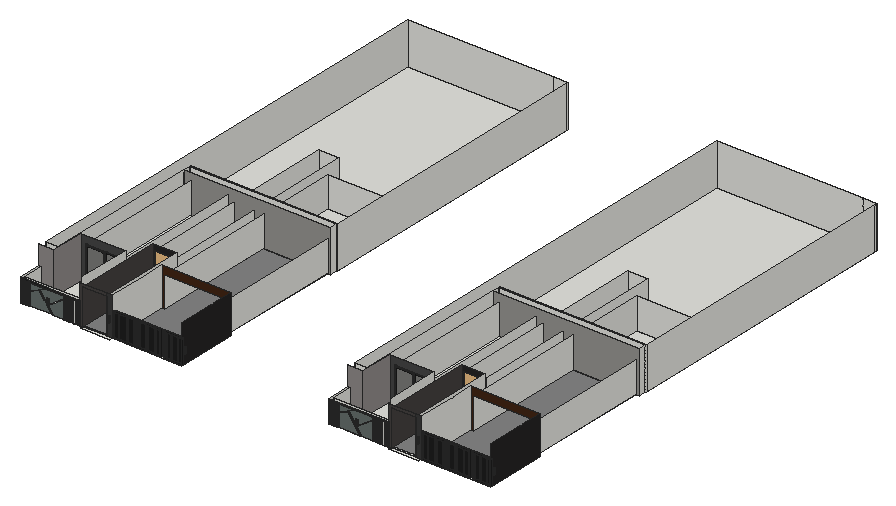
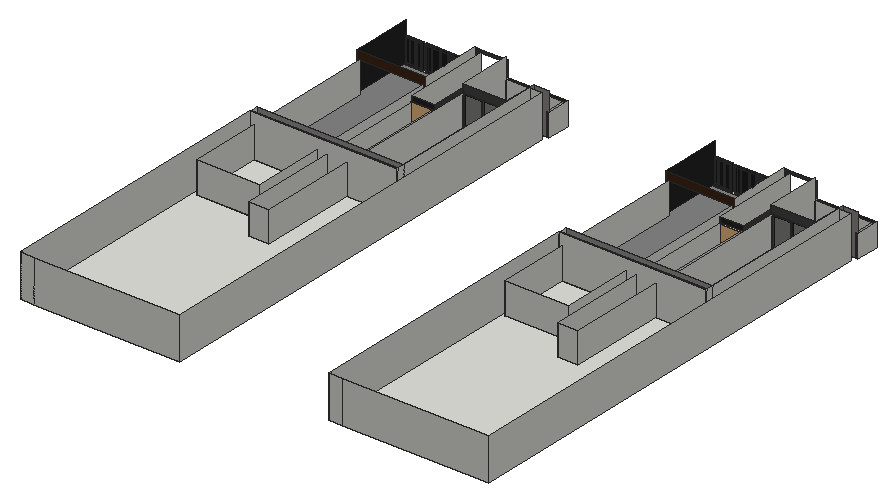
# SketchUp Ruby script. Lengths in inches.
U = 1.inch
M = Sketchup.active_model
def pt(a) = Geom::Point3d.new(a.map { |v| v * U })
def face(e, loops, mat)
  f = e.add_face(loops[0].map { |a| pt(a) })
  loops[1..].each { |l| e.add_face(l.map { |a| pt(a) }).erase! }
  f.material = f.back_material = mat if mat
  f
end
# faces: each face lists its corners as indices into pts; further lists are holes
def faces(e, pts, list, mat = nil) = list.each { |f| face(e, (f[0].is_a?(Array) ? f : [f]).map { |l| l.map { |i| pts[i] } }, mat) }
# xy, xz, yz: faces in a plane at the given z, y or x. An outline is a flat list of corners, or four numbers for a rectangle; further outlines are holes
def ring(l) = l.size == 4 ? [[l[0], l[1]], [l[2], l[1]], [l[2], l[3]], [l[0], l[3]]] : l.each_slice(2).to_a
def flat(e, list, mat, &to3) = list.each { |f| face(e, (f[0].is_a?(Array) ? f : [f]).map { |l| ring(l).map { |u, v| to3.(u, v) } }, mat) }
def xy(e, z, list, mat = nil) = flat(e, list, mat) { |x, y| [x, y, z] }
def xz(e, y, list, mat = nil) = flat(e, list, mat) { |x, z| [x, y, z] }
def yz(e, x, list, mat = nil) = flat(e, list, mat) { |y, z| [x, y, z] }
def lines(e, pts, list) = list.each { |a, b| e.add_line(pt(pts[a]), pt(pts[b])) }
# prism: a flat outline (further loops are holes) pulled along v
def prism(e, loops, v, mat = nil)
  f = face(e, loops, mat); d = Geom::Vector3d.new(v.map { |x| x * U })
  f.pushpull(f.normal.samedirection?(d) ? d.length : -d.length)
end
def box(e, o, s, mat = nil) = prism(e, [[o, [o[0] + s[0], o[1], o[2]], [o[0] + s[0], o[1] + s[1], o[2]], [o[0], o[1] + s[1], o[2]]]], [0, 0, s[2]], mat)
def at(x, y, z, deg = 0) = Geom::Transformation.translation(pt([x, y, z])) * Geom::Transformation.rotation(ORIGIN, Z_AXIS, deg.degrees)
def axes(o, x, y, z) = Geom::Transformation.new([*x, 0, *y, 0, *z, 0, *pt(o).to_a, 1])
def part(name) = M.definitions.add(name)
# library, detail: a bought-in or finely detailed component or shape, given as its bounding box
def library(name, o, s) = part(name).tap { |d| box(d.entities, o, s) }
def detail(e, o, s) = box(e.add_group.entities, o, s)
def put(e, d, t, mat = nil) = e.add_instance(d, t).tap { |i| i.material = mat if mat }
def group(e, t, mat = nil) = e.add_group.tap { |g| g.transformation = t; g.material = mat if mat }.entities
root = M.entities
M.materials.add("Glass_Tinted_Gray").color = [0, 0, 0]
M.materials["Glass_Tinted_Gray"].alpha = 0.125
M.materials.add("[0135_DarkGray]").color = [81, 81, 81]
M.materials.add("[Color M07]").color = [58, 58, 58]
M.materials.add("[Color M08]").color = [30, 30, 30]
M.materials.add("[Granite Dark Gray]").color = [38, 37, 37]
M.materials.add("[Granite Dark Gray]1").color = [69, 68, 68]
M.materials.add("[Granite Light Gray]").color = [149, 148, 144]
M.materials.add("[Granite Tile]1").color = [68, 65, 63]
M.materials.add("[Mirror 02]").color = [229, 229, 229]
M.materials.add("[Slate]").color = [102, 110, 108]
M.materials.add("[Stone Marble]").color = [143, 138, 136]
M.materials.add("[Terrazzo Light Blue]").color = [196, 214, 227]
M.materials.add("[Tile Grey]").color = [132, 132, 132]
M.materials.add("[Wood Veneer 01]").color = [66, 38, 20]
c1 = part("Group\#7")
xy(c1.entities,0,[[6,0,4.45,0.2,3,0.8,1.76,1.76,0.8,3,0.2,4.45,0,6,0.2,7.55,0.8,9,1.76,10.24,3,11.2,4.45,11.8,6,12,7.55,11.8,9,11.2,10.24,10.24,11.2,9,11.8,7.55,12,6,11.8,4.45,11.2,3,10.24,1.76,9,0.8,7.55,0.2]])
xy(c1.entities,37,[[6,0,7.55,0.2,9,0.8,10.24,1.76,11.2,3,11.8,4.45,12,6,11.8,7.55,11.2,9,10.24,10.24,9,11.2,7.55,11.8,6,12,4.45,11.8,3,11.2,1.76,10.24,0.8,9,0.2,7.55,0,6,0.2,4.45,0.8,3,1.76,1.76,3,0.8,4.45,0.2]],"[Granite Tile]1")
p = [[4.45,0.2,0],[6,0,0],[6,0,37],[4.45,0.2,37],[7.55,0.2,0],[7.55,0.2,37],
  [3,0.8,0],[3,0.8,37],[9,0.8,0],[9,0.8,37],[1.76,1.76,0],[1.76,1.76,37],
  [10.24,1.76,0],[10.24,1.76,37],[0.8,3,0],[0.8,3,37],[11.2,3,0],[11.2,3,37],
  [0.2,4.45,0],[0.2,4.45,37],[11.8,4.45,0],[11.8,4.45,37],[0,6,0],[0,6,37],
  [12,6,0],[12,6,37],[0.2,7.55,0],[0.2,7.55,37],[11.8,7.55,0],[11.8,7.55,37],
  [0.8,9,0],[0.8,9,37],[11.2,9,0],[11.2,9,37],[1.76,10.24,0],[1.76,10.24,37],
  [10.24,10.24,0],[10.24,10.24,37],[3,11.2,0],[3,11.2,37],[9,11.2,0],[9,11.2,37],
  [4.45,11.8,0],[4.45,11.8,37],[7.55,11.8,0],[7.55,11.8,37],[6,12,0],[6,12,37]]
faces(c1.entities,p,[[0,1,2,3],[1,4,5,2],[6,0,3,7],[4,8,9,5],[10,6,7,11],[8,12,13,9],[14,10,11,15],[12,16,17,13],
  [18,14,15,19],[16,20,21,17],[22,18,19,23],[20,24,25,21],[26,22,23,27],[24,28,29,25],[30,26,27,31],[28,32,33,29],
  [34,30,31,35],[32,36,37,33],[38,34,35,39],[36,40,41,37],[42,38,39,43],[40,44,45,41],[46,42,43,47],[44,46,47,45]],"[Granite Tile]1")
c2 = part("PENTEK_RP Fineline 50S_Sliding_DoorCase_E1")
box(c2.entities,[0,0,0],[1.51,3.66,99.27],"[0135_DarkGray]")
c3 = part("PENTEK_RP Fineline 50S_SlidingDooe_Case_E2")
box(c3.entities,[0,0,0],[96.25,3.66,1.51],"[0135_DarkGray]")
c4 = part("pentek_RP Fineline 50S_SlidingDoor_Case")
put(c4.entities,c2,at(97.76,0,0))
put(c4.entities,c3,at(1.51,0,0))
put(c4.entities,c2,at(0,0,0))
put(c4.entities,c3,at(1.51,0,97.76))
c5 = part("PENTEK_RP Fineline 50S_SlidingDoor_GlazingBead_2")
box(c5.entities,[0,0,0],[0.56,0.59,94.39],"[0135_DarkGray]")
c6 = part("PENTEK_RP Fineline 50S_SlidingDoor_Glass")
box(c6.entities,[0,0,0],[46.58,0.16,94.39],"Glass_Tinted_Gray")
c7 = part("PENTEK_RP Fineline 50S_SlidingDoor_GlazingBead")
box(c7.entities,[0,0,0],[45.47,0.59,0.56],"[0135_DarkGray]")
c8 = part("PENTEK_RP Fineline 50S_SlidingDoor_Leaf_E1")
xy(c8.entities,0,[[0,0,0.93,1.97],[0.93,1.57,1.49,1.97]],"[0135_DarkGray]")
xy(c8.entities,96.25,[[0,0,0.93,0,0.93,1.57,1.49,1.57,1.49,1.97,0,1.97]],"[0135_DarkGray]")
xz(c8.entities,0,[[0,0,0.93,96.25]],"[0135_DarkGray]")
xz(c8.entities,1.57,[[0.93,0,1.49,95.32],[0.93,95.32,1.49,96.25]],"[0135_DarkGray]")
xz(c8.entities,1.97,[[0,0,1.49,96.25]],"[0135_DarkGray]")
yz(c8.entities,0,[[0,0,1.97,96.25]],"[0135_DarkGray]")
yz(c8.entities,0.93,[[0,0,1.57,0.93],[0,0.93,1.57,95.32],[0,95.32,1.57,96.25]],"[0135_DarkGray]")
yz(c8.entities,1.49,[[1.57,0,1.97,95.32],[1.57,95.32,1.97,96.25]],"[0135_DarkGray]")
c9 = part("PENTEK_RP Fineline 50S_SlidingDoor_Leaf_E2")
xy(c9.entities,0,[[0,0,0,1.57,0.56,1.57,0.56,1.97,46.02,1.97,46.02,1.57,46.58,1.57,46.58,0]],"[0135_DarkGray]")
xy(c9.entities,0.93,[[0,0,46.58,1.57]],"[0135_DarkGray]")
xy(c9.entities,1.49,[[0.56,1.57,46.02,1.97]],"[0135_DarkGray]")
xz(c9.entities,0,[[0,0,46.58,0.93]],"[0135_DarkGray]")
xz(c9.entities,1.57,[[0,0,0.56,0.93],[46.02,0,46.58,0.93],[0.56,0.93,46.02,1.49]],"[0135_DarkGray]")
xz(c9.entities,1.97,[[0.56,0,46.02,1.49]],"[0135_DarkGray]")
yz(c9.entities,0,[[0,0,1.57,0.93]],"[0135_DarkGray]")
yz(c9.entities,0.56,[[1.57,0,1.97,0.93],[1.57,0.93,1.97,1.49]],"[0135_DarkGray]")
yz(c9.entities,46.02,[[1.57,0,1.97,0.93],[1.57,0.93,1.97,1.49]],"[0135_DarkGray]")
yz(c9.entities,46.58,[[0,0,1.57,0.93]],"[0135_DarkGray]")
c10 = part("PENTEK_RP Fineline S_SlidingDoor_Leaf1")
put(c10.entities,c5,at(0.93,0,0.93))
put(c10.entities,c5,at(46.96,0,0.93))
put(c10.entities,c6,at(1.49,1.42,0.93))
put(c10.entities,c7,at(1.49,0,0.93))
put(c10.entities,c6,at(1.49,0.59,0.93),"[Terrazzo Light Blue]")
put(c10.entities,c8,at(0,0,0))
put(c10.entities,c8,axes([48.44,0,0],[-1,0,0],[0,1,0],[0,0,1]))
put(c10.entities,c9,axes([0.93,0,96.25],[1,0,0],[0,1,0],[0,0,-1]))
put(c10.entities,c9,at(0.93,0,0))
put(c10.entities,c7,at(1.49,0,94.77))
c11 = part("PENTEK_RP Fineline 50S_SlidingDoor_Leaf2")
put(c11.entities,c6,at(1.49,1.42,0.93))
put(c11.entities,c7,at(1.49,0,94.77))
put(c11.entities,c5,at(46.96,0,0.93))
put(c11.entities,c6,at(1.49,0.59,0.93),"[Mirror 02]")
put(c11.entities,c5,at(0.93,0,0.93))
put(c11.entities,c8,at(0,0,0))
put(c11.entities,c8,axes([48.44,0,0],[-1,0,0],[0,1,0],[0,0,1]))
put(c11.entities,c7,at(1.49,0,0.93))
put(c11.entities,c9,axes([0.93,0,96.25],[1,0,0],[0,1,0],[0,0,-1]))
put(c11.entities,c9,at(0.93,0,0))
c12 = part("PENTEK - Slimmest Steel Sliding Door / Window\#1")
put(c12.entities,c4,at(0,-1.88,-0.09))
put(c12.entities,c10,at(1.51,-2.27,1.42))
put(c12.entities,c11,at(49.32,-0.3,1.42))
c13 = library("元件\#5",[-4.39,0,0],[5.37,35.83,90.55])
c14 = part("Group\#102")
g1 = group(c14.entities,at(0,0,0))
prism(g1,[[[0,3,72],[70.5,3,72],[70.5,3,0],[0,3,0]],[[67.5,3,3],[67.5,3,69],[3,3,69],[3,3,3]]],[0,-3,0])
c15 = part("Group\#135")
box(c15.entities,[0,0,0],[0.5,1,66])
c16 = part("Group\#148")
box(c16.entities,[0,-1,0],[5.5,1,66])
box(c16.entities,[50.84,-1,0],[13.66,1,66])
box(c16.entities,[28.06,-1,0],[22.28,1,66])
box(c16.entities,[24.66,-1,0],[2.9,1,66])
box(c16.entities,[6,-1,0],[18.16,1,66])
c17 = part("Component\#23")
g2 = group(c17.entities,at(70.5,0,0),"[Color M08]")
put(g2,c14,axes([70.5,0,0],[-1,0,0],[0,1,0],[0,0,1]))
g3 = group(g2,at(3,2,3))
g4 = group(g3,at(0,-1,0))
box(g4,[0,0,0],[5.5,1,66])
box(g4,[50.84,0,0],[13.66,1,66])
box(g4,[28.06,0,0],[22.28,1,66])
box(g4,[24.66,0,0],[2.9,1,66])
box(g4,[6,0,0],[18.16,1,66])
put(g3,c15,axes([50.34,0,0],[1,0,0],[0,-1,0],[0,0,1]))
put(g3,c15,axes([24.16,0,0],[1,0,0],[0,-1,0],[0,0,1]))
put(g3,c15,axes([27.56,0,0],[1,0,0],[0,-1,0],[0,0,1]))
put(g3,c15,axes([5.5,0,0],[1,0,0],[0,-1,0],[0,0,1]))
g5 = group(c17.entities,at(70.5,0,0),"[Color M08]")
put(g5,c14,at(-70.5,0,0))
g6 = group(g5,at(-3,2,3,-180))
put(g6,c16,at(0,1,0))
put(g6,c15,at(50.34,0,0))
put(g6,c15,at(24.16,0,0))
put(g6,c15,at(27.56,0,0))
put(g6,c15,at(5.5,0,0))
g7 = group(c17.entities,at(150,0,0),"[Color M08]")
put(g7,c14,axes([54,0,0],[-0.76596,0,0],[0,1,0],[0,0,1]))
g8 = group(g7,at(2.3,2,3))
put(g8,c16,axes([0,-1,0],[0.76596,0,0],[0,-1,0],[0,0,1]))
put(g8,c15,axes([38.55,0,0],[0.76596,0,0],[0,-1,0],[0,0,1]))
put(g8,c15,axes([18.5,0,0],[0.76596,0,0],[0,-1,0],[0,0,1]))
put(g8,c15,axes([21.11,0,0],[0.76596,0,0],[0,-1,0],[0,0,1]))
put(g8,c15,axes([4.22,0,0],[0.76596,0,0],[0,-1,0],[0,0,1]))
xy(root,8.5,[[2153.45,450,2237.65,458.5],[3032.2,450,3116.4,458.5],[1976.47,457.5625,1980.03,458.5],[1981.28,457.5625,1984.84,458.5],[1986.1,457.5625,1989.66,458.5],
  [1990.91,457.5625,1994.47,458.5],[1995.72,457.5625,1999.28,458.5],[2000.53,457.5625,2004.09,458.5],[2100.97,457.5625,2104.93,458.5],[2105.97,457.5625,2109.93,458.5],
  [2110.97,457.5625,2114.93,458.5],[2115.97,457.5625,2119.93,458.5],[2120.97,457.5625,2124.93,458.5],[2125.97,457.5625,2129.93,458.5],[2135.7,457.5625,2139.36,458.5],
  [2143.16,457.5625,2146.28,458.5],[2855.22,457.5625,2858.78,458.5],[2860.03,457.5625,2863.59,458.5],[2864.85,457.5625,2868.41,458.5],[2869.66,457.5625,2873.22,458.5],
  [2874.47,457.5625,2878.03,458.5],[2879.28,457.5625,2882.84,458.5],[2979.72,457.5625,2983.68,458.5],[2984.72,457.5625,2988.68,458.5],[2989.72,457.5625,2993.68,458.5],
  [2994.72,457.5625,2998.68,458.5],[2999.72,457.5625,3003.68,458.5],[3004.72,457.5625,3008.68,458.5],[3014.45,457.5625,3018.11,458.5],[3021.91,457.5625,3025.03,458.5],
  [1976.47,458.5,1976.47,523.18,1983.29,523.18,1983.29,465.32,2146.28,465.32,2146.28,458.5,2067.62,458.5,2067.62,461.375,2064.07,461.375,2064.07,458.5],[2064.07,458.5,2067.62,461.375],[2153.45,458.5,2221.2,465.32],[2238.79,458.5,2436.4,465.32],[2855.22,458.5,2855.22,523.18,2862.04,523.18,2862.04,465.32,3025.03,465.32,3025.03,458.5,2946.37,458.5,2946.37,461.375,2942.82,461.375,2942.82,458.5],
  [2942.82,458.5,2946.37,461.375],[3032.2,458.5,3099.95,465.32],[3117.54,458.5,3315.15,465.32],[1983.29,465.32,2146.28,465.32,2146.28,619.06,2020.16,619.06,2020.16,523.18,1983.29,523.18],[2862.04,465.32,3025.03,465.32,3025.03,619.06,2898.91,619.06,2898.91,523.18,2862.04,523.18],
  [1983.29,539.02,2019.03,539.02,2019.03,1010.9,2160.47,1010.9,2160.47,1288.43,2218.35,1288.43,2218.35,1010.9,2246.4,1010.9,2246.4,1213.68,2427.3,1213.68,2427.3,1010.9,2436.4,1010.9,2436.4,1828.81,1983.29,1828.81],[2862.04,539.02,2897.78,539.02,2897.78,1010.9,3039.22,1010.9,3039.22,1288.43,3097.1,1288.43,3097.1,1010.9,3125.15,1010.9,3125.15,1213.68,3306.05,1213.68,3306.05,1010.9,3315.15,1010.9,3315.15,1828.81,2862.04,1828.81],[2019.03,986.46,2160.47,1006.15],[2160.47,986.46,2218.35,1006.15],[2218.35,986.46,2246.4,1006.15],
  [2246.4,986.46,2427.3,1006.15],[2427.3,986.46,2436.4,1006.15],[2897.78,986.46,3039.22,1006.15],[3039.22,986.46,3097.1,1006.15],[3097.1,986.46,3125.15,1006.15],
  [3125.15,986.46,3306.05,1006.15],[3306.05,986.46,3315.15,1006.15],[2019.03,1006.15,2160.47,1010.9],[2160.47,1006.15,2218.35,1010.9],[2218.35,1006.15,2246.4,1010.9],
  [2246.4,1006.15,2427.3,1010.9],[2427.3,1006.15,2436.4,1010.9],[2897.78,1006.15,3039.22,1010.9],[3039.22,1006.15,3097.1,1010.9],[3097.1,1006.15,3125.15,1010.9],
  [3125.15,1006.15,3306.05,1010.9],[3306.05,1006.15,3315.15,1010.9],[2160.47,1010.9,2218.35,1288.43],[2246.4,1010.9,2427.3,1213.68],[3039.22,1010.9,3097.1,1288.43],
  [3125.15,1010.9,3306.05,1213.68]])
xy(root,8.5,[[2153.45,465.32,2221.2,465.32,2221.2,706.62,2218.35,706.62,2218.35,986.46,2160.47,986.46,2160.47,706.62,2153.45,706.62],[2238.79,465.32,2436.4,465.32,2436.4,633.06,2427.3,633.06,2427.3,986.46,2246.4,986.46,2246.4,633.06,2238.79,633.06],[3032.2,465.32,3099.95,465.32,3099.95,706.62,3097.1,706.62,3097.1,986.46,3039.22,986.46,3039.22,706.62,3032.2,706.62],[3117.54,465.32,3315.15,465.32,3315.15,633.06,3306.05,633.06,3306.05,986.46,3125.15,986.46,3125.15,633.06,3117.54,633.06]],"[Tile Grey]")
xy(root,20.01,[[2037.38,619.06,2142.51,1006.15],[2916.13,619.06,3021.26,1006.15]])
xy(root,68.78,[[1980.03,457.5625,1981.28,458.5],[1984.84,457.5625,1986.1,458.5],[1989.66,457.5625,1990.91,458.5],[1994.47,457.5625,1995.72,458.5],[1999.28,457.5625,2000.53,458.5],
  [2004.09,457.5625,2004.09,458.5,2047.85,458.5,2047.85,461.375,2050.98,461.375,2050.98,458.5,2100.97,458.5,2100.97,457.5625],[2104.93,457.5625,2105.97,458.5],[2109.93,457.5625,2110.97,458.5],[2114.93,457.5625,2115.97,458.5],[2119.93,457.5625,2120.97,458.5],
  [2124.93,457.5625,2125.97,458.5],[2129.93,457.5625,2135.7,458.5],[2139.36,457.5625,2143.16,458.5],[2858.78,457.5625,2860.03,458.5],[2863.59,457.5625,2864.85,458.5],
  [2868.41,457.5625,2869.66,458.5],[2873.22,457.5625,2874.47,458.5],[2878.03,457.5625,2879.28,458.5],[2882.84,457.5625,2882.84,458.5,2926.6,458.5,2926.6,461.375,2929.73,461.375,2929.73,458.5,2979.72,458.5,2979.72,457.5625],[2983.68,457.5625,2984.72,458.5],
  [2988.68,457.5625,2989.72,458.5],[2993.68,457.5625,2994.72,458.5],[2998.68,457.5625,2999.72,458.5],[3003.68,457.5625,3004.72,458.5],[3008.68,457.5625,3014.45,458.5],
  [3018.11,457.5625,3021.91,458.5]])
xz(root,457.5625,[[1976.47,8.5,1980.03,68.78],[1981.28,8.5,1984.84,68.78],[1986.1,8.5,1989.66,68.78],[1990.91,8.5,1994.47,68.78],[1995.72,8.5,1999.28,68.78],
  [2000.53,8.5,2004.09,68.78],[2100.97,8.5,2104.93,68.78],[2105.97,8.5,2109.93,68.78],[2110.97,8.5,2114.93,68.78],[2115.97,8.5,2119.93,68.78],
  [2120.97,8.5,2124.93,68.78],[2143.16,8.5,2146.28,68.78],[2855.22,8.5,2858.78,68.78],[2860.03,8.5,2863.59,68.78],[2864.85,8.5,2868.41,68.78],
  [2869.66,8.5,2873.22,68.78],[2874.47,8.5,2878.03,68.78],[2879.28,8.5,2882.84,68.78],[2979.72,8.5,2983.68,68.78],[2984.72,8.5,2988.68,68.78],
  [2989.72,8.5,2993.68,68.78],[2994.72,8.5,2998.68,68.78],[2999.72,8.5,3003.68,68.78],[3021.91,8.5,3025.03,68.78],[1976.47,68.78,2146.28,72.4375],
  [2855.22,68.78,3025.03,72.4375]],"[Color M08]")
xz(root,457.5625,[[2125.97,8.5,2129.93,68.78],[2135.7,8.5,2139.36,68.78],[3004.72,8.5,3008.68,68.78],[3014.45,8.5,3018.11,68.78]],"[Slate]")
xz(root,458.5,[[1980.03,8.5,1981.28,68.78],[1984.84,8.5,1986.1,68.78],[1989.66,8.5,1990.91,68.78],[1994.47,8.5,1995.72,68.78],[1999.28,8.5,2000.53,68.78],
  [2104.93,8.5,2105.97,68.78],[2109.93,8.5,2110.97,68.78],[2114.93,8.5,2115.97,68.78],[2119.93,8.5,2120.97,68.78],[2124.93,8.5,2125.97,68.78],
  [2858.78,8.5,2860.03,68.78],[2863.59,8.5,2864.85,68.78],[2868.41,8.5,2869.66,68.78],[2873.22,8.5,2874.47,68.78],[2878.03,8.5,2879.28,68.78],
  [2983.68,8.5,2984.72,68.78],[2988.68,8.5,2989.72,68.78],[2993.68,8.5,2994.72,68.78],[2998.68,8.5,2999.72,68.78],[3003.68,8.5,3004.72,68.78]])
xz(root,458.5,[[2221.2,8.5,2238.79,118.38],[3099.95,8.5,3117.54,118.38]],"[Color M07]")
xz(root,458.5,[[2129.93,8.5,2135.7,68.78],[2139.36,8.5,2143.16,68.78],[3008.68,8.5,3014.45,68.78],[3018.11,8.5,3021.91,68.78]],"[Color M08]")
xz(root,458.5,[[2146.28,8.5,2153.45,8.5,2153.45,110.32,2221.2,110.32,2221.2,118.38,2146.28,118.38],[3025.03,8.5,3032.2,8.5,3032.2,110.32,3099.95,110.32,3099.95,118.38,3025.03,118.38]],"[Granite Tile]1")
xz(root,458.5,[[2004.09,8.5,2064.07,8.5,2029.37,57.375,2004.09,44.04],[2067.62,8.5,2100.97,8.5,2100.97,58.8,2055.31,25.91],[2882.84,8.5,2942.82,8.5,2908.12,57.375,2882.84,44.04],[2946.37,8.5,2979.72,8.5,2979.72,58.8,2934.06,25.91],[2052.89,29.34,2100.97,62.06,2100.97,68.78,2050.98,68.78,2032.07,58.8],
  [2931.64,29.34,2979.72,62.06,2979.72,68.78,2929.73,68.78,2910.82,58.8],[2004.09,46.32,2047.85,68.78,2004.09,68.78],[2882.84,46.32,2926.6,68.78,2882.84,68.78]],"[Slate]")
xz(root,461.375,[[2064.07,8.5,2067.62,8.5,2055.31,25.91,2052.89,29.34,2032.07,58.8,2029.37,57.375],[2942.82,8.5,2946.37,8.5,2934.06,25.91,2931.64,29.34,2910.82,58.8,2908.12,57.375],[2055.31,25.91,2100.97,58.8,2100.97,62.06,2052.89,29.34],[2934.06,25.91,2979.72,58.8,2979.72,62.06,2931.64,29.34],[2004.09,44.04,2029.37,57.375,2032.07,58.8,2050.98,68.78,2047.85,68.78,2004.09,46.32],
  [2882.84,44.04,2908.12,57.375,2910.82,58.8,2929.73,68.78,2926.6,68.78,2882.84,46.32]])
xz(root,465.32,[[1983.29,8.5,2146.28,72.4375],[2862.04,8.5,3025.03,72.4375]])
xz(root,523.18,[[1976.47,8.5,1983.29,72.4375],[2855.22,8.5,2862.04,72.4375]])
xz(root,523.18,[[1983.29,8.5,2020.16,8.5,2020.16,128.5,1976.47,128.5,1976.47,72.4375,1983.29,72.4375],[2862.04,8.5,2898.91,8.5,2898.91,128.5,2855.22,128.5,2855.22,72.4375,2862.04,72.4375]],"[Stone Marble]")
xz(root,539.02,[[1983.29,8.5,2019.03,128.5],[2862.04,8.5,2897.78,128.5]])
xz(root,619.06,[[[2020.16,8.5,2146.28,128.5],[2037.38,20.01,2142.51,107.07]],[[2898.91,8.5,3025.03,128.5],[2916.13,20.01,3021.26,107.07]]],"[Granite Dark Gray]1")
xz(root,633.06,[[2238.79,8.5,2246.4,8.5,2246.4,96.29,2427.3,96.29,2427.3,8.5,2436.4,8.5,2436.4,118.38,2238.79,118.38],[3117.54,8.5,3125.15,8.5,3125.15,96.29,3306.05,96.29,3306.05,8.5,3315.15,8.5,3315.15,118.38,3117.54,118.38]],"[Wood Veneer 01]")
xz(root,706.62,[[2153.45,8.5,2160.47,8.5,2160.47,96.1875,2218.35,96.1875,2218.35,8.5,2221.2,8.5,2221.2,110.32,2153.45,110.32],[3032.2,8.5,3039.22,8.5,3039.22,96.1875,3097.1,96.1875,3097.1,8.5,3099.95,8.5,3099.95,110.32,3032.2,110.32]],"[Granite Dark Gray]")
xz(root,986.46,[[2019.03,8.5,2436.4,128.5],[2897.78,8.5,3315.15,128.5]],"[Granite Light Gray]")
xz(root,1006.15,[[[2019.03,8.5,2436.4,128.5],[2037.38,20.01,2142.51,107.07]],[[2897.78,8.5,3315.15,128.5],[2916.13,20.01,3021.26,107.07]]])
xz(root,1010.9,[[2019.03,8.5,2436.4,128.5],[2897.78,8.5,3315.15,128.5]])
xz(root,1213.68,[[2246.4,8.5,2427.3,96.29],[3125.15,8.5,3306.05,96.29]])
xz(root,1288.43,[[2160.47,8.5,2218.35,96.1875],[3039.22,8.5,3097.1,96.1875]])
xz(root,1828.81,[[1983.29,8.5,2397.9,128.5],[2397.9,8.5,2436.4,128.5],[2862.04,8.5,3276.65,128.5],[3276.65,8.5,3315.15,128.5]])
yz(root,1976.47,[[457.5625,8.5,523.18,72.4375]])
yz(root,1980.03,[[457.5625,8.5,458.5,68.78]])
yz(root,1981.28,[[457.5625,8.5,458.5,68.78]])
yz(root,1983.29,[[465.32,8.5,523.18,72.4375],[539.02,8.5,1828.81,128.5]])
yz(root,1984.84,[[457.5625,8.5,458.5,68.78]])
yz(root,1986.1,[[457.5625,8.5,458.5,68.78]])
yz(root,1989.66,[[457.5625,8.5,458.5,68.78]])
yz(root,1990.91,[[457.5625,8.5,458.5,68.78]])
yz(root,1994.47,[[457.5625,8.5,458.5,68.78]])
yz(root,1995.72,[[457.5625,8.5,458.5,68.78]])
yz(root,1999.28,[[457.5625,8.5,458.5,68.78]])
yz(root,2000.53,[[457.5625,8.5,458.5,68.78]])
yz(root,2004.09,[[457.5625,8.5,458.5,8.5,458.5,44.04,461.375,44.04,461.375,46.32,458.5,46.32,458.5,68.78,457.5625,68.78]])
yz(root,2019.03,[[539.02,8.5,986.46,128.5],[986.46,8.5,1006.15,128.5],[1006.15,8.5,1010.9,128.5]])
yz(root,2020.16,[[523.18,8.5,619.06,128.5]],"[Stone Marble]")
yz(root,2037.38,[[619.06,20.01,1006.15,107.07]])
yz(root,2100.97,[[457.5625,8.5,457.5625,68.78,458.5,68.78,458.5,62.06,461.375,62.06,461.375,58.8,458.5,58.8,458.5,8.5]])
yz(root,2104.93,[[457.5625,8.5,458.5,68.78]])
yz(root,2105.97,[[457.5625,8.5,458.5,68.78]])
yz(root,2109.93,[[457.5625,8.5,458.5,68.78]])
yz(root,2110.97,[[457.5625,8.5,458.5,68.78]])
yz(root,2114.93,[[457.5625,8.5,458.5,68.78]])
yz(root,2115.97,[[457.5625,8.5,458.5,68.78]])
yz(root,2119.93,[[457.5625,8.5,458.5,68.78]])
yz(root,2120.97,[[457.5625,8.5,458.5,68.78]])
yz(root,2124.93,[[457.5625,8.5,458.5,68.78]])
yz(root,2125.97,[[457.5625,8.5,458.5,68.78]])
yz(root,2129.93,[[457.5625,8.5,458.5,68.78]])
yz(root,2135.7,[[457.5625,8.5,458.5,68.78]])
yz(root,2139.36,[[457.5625,8.5,458.5,68.78]])
yz(root,2142.51,[[619.06,20.01,1006.15,107.07]])
yz(root,2143.16,[[457.5625,8.5,458.5,68.78]])
yz(root,2146.28,[[457.5625,8.5,458.5,68.78],[458.5,8.5,465.32,72.4375],[465.32,8.5,619.06,128.5],[457.5625,68.78,458.5,72.4375]])
yz(root,2153.45,[[458.5,8.5,706.62,110.32]],"[Granite Tile]1")
yz(root,2160.47,[[706.62,8.5,1288.43,96.1875]])
yz(root,2218.35,[[706.62,8.5,1288.43,96.1875]])
yz(root,2221.2,[[458.5,8.5,706.62,110.32]])
yz(root,2238.79,[[458.5,8.5,633.06,8.5,633.06,118.38,571.64,118.38,571.64,116.94,561.06,116.94,561.06,118.38,458.5,118.38]])
yz(root,2246.4,[[633.06,8.5,1213.68,96.29]])
yz(root,2427.3,[[633.06,8.5,1213.68,96.29]])
yz(root,2436.4,[[986.46,8.5,1006.15,128.5],[1006.15,8.5,1010.9,128.5],[1010.9,8.5,1822.82,128.5],[1822.82,8.5,1828.81,128.5]])
yz(root,2436.4,[[458.5,8.5,458.5,118.38,561.06,118.38,561.06,116.94,571.64,116.94,571.64,118.38,633.06,118.38,633.06,8.5]],"[Granite Dark Gray]")
yz(root,2855.22,[[457.5625,8.5,523.18,72.4375]])
yz(root,2858.78,[[457.5625,8.5,458.5,68.78]])
yz(root,2860.03,[[457.5625,8.5,458.5,68.78]])
yz(root,2862.04,[[465.32,8.5,523.18,72.4375],[539.02,8.5,1828.81,128.5]])
yz(root,2863.59,[[457.5625,8.5,458.5,68.78]])
yz(root,2864.85,[[457.5625,8.5,458.5,68.78]])
yz(root,2868.41,[[457.5625,8.5,458.5,68.78]])
yz(root,2869.66,[[457.5625,8.5,458.5,68.78]])
yz(root,2873.22,[[457.5625,8.5,458.5,68.78]])
yz(root,2874.47,[[457.5625,8.5,458.5,68.78]])
yz(root,2878.03,[[457.5625,8.5,458.5,68.78]])
yz(root,2879.28,[[457.5625,8.5,458.5,68.78]])
yz(root,2882.84,[[457.5625,8.5,458.5,8.5,458.5,44.04,461.375,44.04,461.375,46.32,458.5,46.32,458.5,68.78,457.5625,68.78]])
yz(root,2897.78,[[539.02,8.5,986.46,128.5],[986.46,8.5,1006.15,128.5],[1006.15,8.5,1010.9,128.5]])
yz(root,2898.91,[[523.18,8.5,619.06,128.5]],"[Stone Marble]")
yz(root,2916.13,[[619.06,20.01,1006.15,107.07]])
yz(root,2979.72,[[457.5625,8.5,457.5625,68.78,458.5,68.78,458.5,62.06,461.375,62.06,461.375,58.8,458.5,58.8,458.5,8.5]])
yz(root,2983.68,[[457.5625,8.5,458.5,68.78]])
yz(root,2984.72,[[457.5625,8.5,458.5,68.78]])
yz(root,2988.68,[[457.5625,8.5,458.5,68.78]])
yz(root,2989.72,[[457.5625,8.5,458.5,68.78]])
yz(root,2993.68,[[457.5625,8.5,458.5,68.78]])
yz(root,2994.72,[[457.5625,8.5,458.5,68.78]])
yz(root,2998.68,[[457.5625,8.5,458.5,68.78]])
yz(root,2999.72,[[457.5625,8.5,458.5,68.78]])
yz(root,3003.68,[[457.5625,8.5,458.5,68.78]])
yz(root,3004.72,[[457.5625,8.5,458.5,68.78]])
yz(root,3008.68,[[457.5625,8.5,458.5,68.78]])
yz(root,3014.45,[[457.5625,8.5,458.5,68.78]])
yz(root,3018.11,[[457.5625,8.5,458.5,68.78]])
yz(root,3021.26,[[619.06,20.01,1006.15,107.07]])
yz(root,3021.91,[[457.5625,8.5,458.5,68.78]])
yz(root,3025.03,[[457.5625,8.5,458.5,68.78],[458.5,8.5,465.32,72.4375],[465.32,8.5,619.06,128.5],[457.5625,68.78,458.5,72.4375]])
yz(root,3032.2,[[458.5,8.5,706.62,110.32]],"[Granite Tile]1")
yz(root,3039.22,[[706.62,8.5,1288.43,96.1875]])
yz(root,3097.1,[[706.62,8.5,1288.43,96.1875]])
yz(root,3099.95,[[458.5,8.5,706.62,110.32]])
yz(root,3117.54,[[458.5,8.5,633.06,8.5,633.06,118.38,571.64,118.38,571.64,116.94,561.06,116.94,561.06,118.38,458.5,118.38]])
yz(root,3125.15,[[633.06,8.5,1213.68,96.29]])
yz(root,3306.05,[[633.06,8.5,1213.68,96.29]])
yz(root,3315.15,[[986.46,8.5,1006.15,128.5],[1006.15,8.5,1010.9,128.5],[1010.9,8.5,1822.82,128.5],[1822.82,8.5,1828.81,128.5]])
yz(root,3315.15,[[458.5,8.5,458.5,118.38,561.06,118.38,561.06,116.94,571.64,116.94,571.64,118.38,633.06,118.38,633.06,8.5]],"[Granite Dark Gray]")
p = [[2029.37,458.5,57.375],[2064.07,458.5,8.5],[2064.07,461.375,8.5],[2029.37,461.375,57.375],[2067.62,458.5,8.5],[2055.31,458.5,25.91],
  [2055.31,461.375,25.91],[2067.62,461.375,8.5],[2908.12,458.5,57.375],[2942.82,458.5,8.5],[2942.82,461.375,8.5],[2908.12,461.375,57.375],
  [2946.37,458.5,8.5],[2934.06,458.5,25.91],[2934.06,461.375,25.91],[2946.37,461.375,8.5],[2100.97,458.5,58.8],[2100.97,461.375,58.8],
  [2979.72,458.5,58.8],[2979.72,461.375,58.8],[2052.89,458.5,29.34],[2032.07,458.5,58.8],[2032.07,461.375,58.8],[2052.89,461.375,29.34],
  [2100.97,458.5,62.06],[2100.97,461.375,62.06],[2931.64,458.5,29.34],[2910.82,458.5,58.8],[2910.82,461.375,58.8],[2931.64,461.375,29.34],
  [2979.72,458.5,62.06],[2979.72,461.375,62.06],[2004.09,458.5,44.04],[2004.09,461.375,44.04],[2882.84,458.5,44.04],[2882.84,461.375,44.04],
  [2047.85,458.5,68.78],[2004.09,458.5,46.32],[2004.09,461.375,46.32],[2047.85,461.375,68.78],[2926.6,458.5,68.78],[2882.84,458.5,46.32],
  [2882.84,461.375,46.32],[2926.6,461.375,68.78],[2050.98,458.5,68.78],[2050.98,461.375,68.78],[2929.73,458.5,68.78],[2929.73,461.375,68.78]]
faces(root,p,[[0,1,2,3],[4,5,6,7],[8,9,10,11],[12,13,14,15],[5,16,17,6],[13,18,19,14],[20,21,22,23],[24,20,23,25],
  [26,27,28,29],[30,26,29,31],[32,0,3,33],[34,8,11,35],[36,37,38,39],[40,41,42,43],[21,44,45,22],[27,46,47,28]])
put(root,c1,axes([2051.85,456.34,29.51],[0.42,0,0],[0,0.42,0],[0,0,0.42]))
put(root,c12,axes([2034.38,619.06,20],[1.08916,0,0],[0,1,0],[0,0,0.87793]))
put(root,c13,axes([2160.47,706.99,8.5],[0,-1,0],[1.61541,0,0],[0,0,0.96838]))
put(root,c1,axes([2227.28,453.46,47.16],[0.42,0,0],[0,0.42,0],[0,0,0.42]))
put(root,c17,axes([2238.79,458.5,8.5],[0.9687,0,0],[0,1,0],[0,0,1]))
put(root,c1,axes([2443.36,453.46,44.5],[0.42,0,0],[0,0.42,0],[0,0,0.42]))
put(root,c1,axes([2930.6,456.34,29.51],[0.42,0,0],[0,0.42,0],[0,0,0.42]))
put(root,c12,axes([2913.13,619.06,20],[1.08916,0,0],[0,1,0],[0,0,0.87793]))
put(root,c13,axes([3039.22,706.99,8.5],[0,-1,0],[1.61541,0,0],[0,0,0.96838]))
put(root,c1,axes([3106.03,453.46,47.16],[0.42,0,0],[0,0.42,0],[0,0,0.42]))
put(root,c17,axes([3117.54,458.5,8.5],[0.9687,0,0],[0,1,0],[0,0,1]))
put(root,c1,axes([3322.11,453.46,44.5],[0.42,0,0],[0,0.42,0],[0,0,0.42]))
